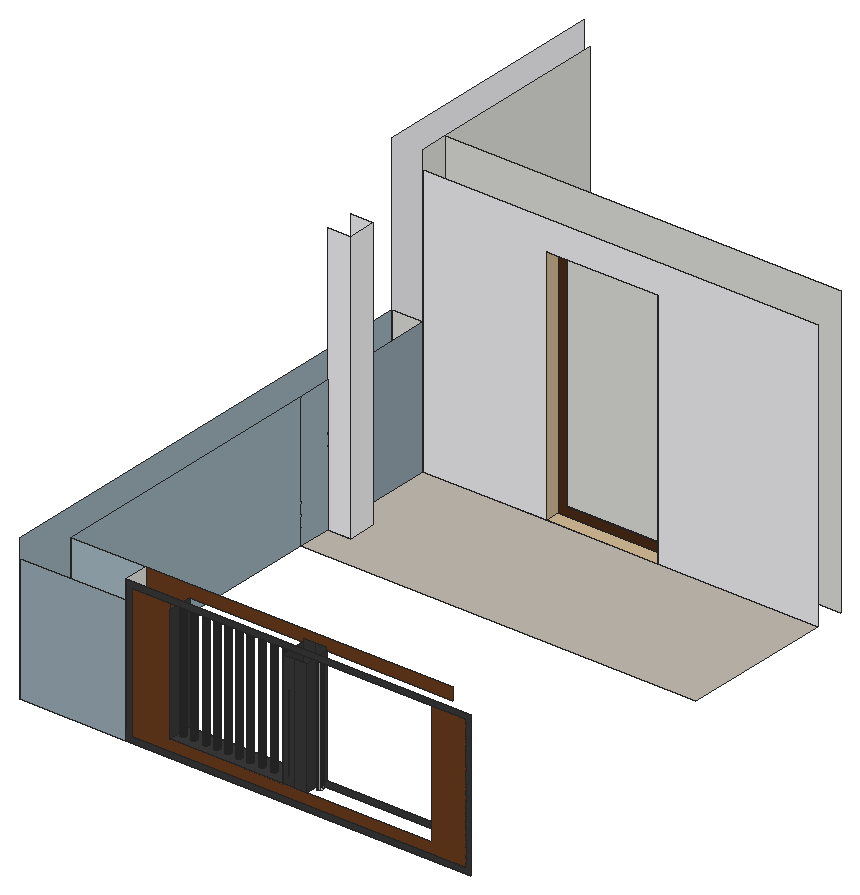
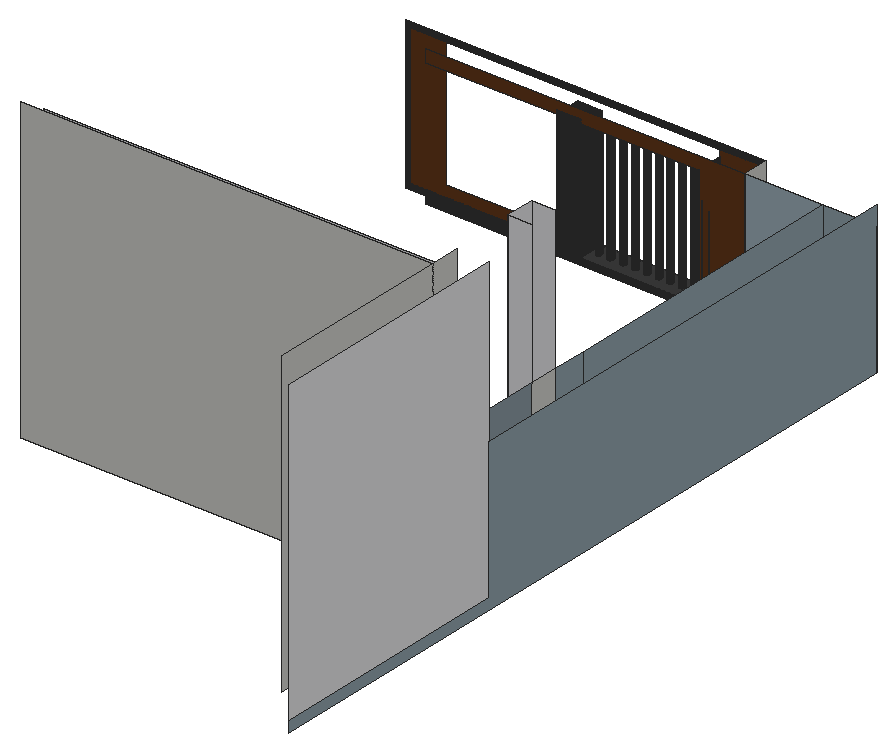
# SketchUp Ruby script. Lengths in inches.
U = 1.inch
M = Sketchup.active_model
def pt(a) = Geom::Point3d.new(a.map { |v| v * U })
def face(e, loops, mat)
  f = e.add_face(loops[0].map { |a| pt(a) })
  loops[1..].each { |l| e.add_face(l.map { |a| pt(a) }).erase! }
  f.material = f.back_material = mat if mat
  f
end
# faces: each face lists its corners as indices into pts; further lists are holes
def faces(e, pts, list, mat = nil) = list.each { |f| face(e, (f[0].is_a?(Array) ? f : [f]).map { |l| l.map { |i| pts[i] } }, mat) }
# xy, xz, yz: faces in a plane at the given z, y or x. An outline is a flat list of corners, or four numbers for a rectangle; further outlines are holes
def ring(l) = l.size == 4 ? [[l[0], l[1]], [l[2], l[1]], [l[2], l[3]], [l[0], l[3]]] : l.each_slice(2).to_a
def flat(e, list, mat, &to3) = list.each { |f| face(e, (f[0].is_a?(Array) ? f : [f]).map { |l| ring(l).map { |u, v| to3.(u, v) } }, mat) }
def xy(e, z, list, mat = nil) = flat(e, list, mat) { |x, y| [x, y, z] }
def xz(e, y, list, mat = nil) = flat(e, list, mat) { |x, z| [x, y, z] }
def yz(e, x, list, mat = nil) = flat(e, list, mat) { |y, z| [x, y, z] }
def lines(e, pts, list) = list.each { |a, b| e.add_line(pt(pts[a]), pt(pts[b])) }
# prism: a flat outline (further loops are holes) pulled along v
def prism(e, loops, v, mat = nil)
  f = face(e, loops, mat); d = Geom::Vector3d.new(v.map { |x| x * U })
  f.pushpull(f.normal.samedirection?(d) ? d.length : -d.length)
end
def box(e, o, s, mat = nil) = prism(e, [[o, [o[0] + s[0], o[1], o[2]], [o[0] + s[0], o[1] + s[1], o[2]], [o[0], o[1] + s[1], o[2]]]], [0, 0, s[2]], mat)
def at(x, y, z, deg = 0) = Geom::Transformation.translation(pt([x, y, z])) * Geom::Transformation.rotation(ORIGIN, Z_AXIS, deg.degrees)
def axes(o, x, y, z) = Geom::Transformation.new([*x, 0, *y, 0, *z, 0, *pt(o).to_a, 1])
def part(name) = M.definitions.add(name)
# library, detail: a bought-in or finely detailed component or shape, given as its bounding box
def library(name, o, s) = part(name).tap { |d| box(d.entities, o, s) }
def detail(e, o, s) = box(e.add_group.entities, o, s)
def put(e, d, t, mat = nil) = e.add_instance(d, t).tap { |i| i.material = mat if mat }
def group(e, t, mat = nil) = e.add_group.tap { |g| g.transformation = t; g.material = mat if mat }.entities
root = M.entities
M.materials.add("[Blinds Vertical Pattern]").color = [245, 245, 247]
M.materials.add("[Blinds Vertical Pattern]3").color = [247, 247, 249]
M.materials.add("[Color M03]").color = [170, 170, 170]
M.materials.add("[Color M07]").color = [58, 58, 58]
M.materials.add("[Field Rectangle Tile]").color = [196, 189, 179]
M.materials.add("[Formica Beige]").color = [211, 187, 149]
M.materials.add("[Formica Speckled Grey]").color = [157, 176, 186]
M.materials.add("[Formica Speckled Grey]1").color = [149, 166, 175]
M.materials.add("[Formica Speckled Grey]2").color = [170, 190, 201]
M.materials.add("[Wood Cherry Original]").color = [107, 60, 29]
M.materials.add("[Wood Veneer 01]").color = [76, 44, 23]
xy(root,9,[[62.71,489.78,81.96,513.87]])
xy(root,9,[[62.71,461.03,399.08,461.03,399.08,590.55,62.71,590.55,62.71,513.87,81.96,513.87,81.96,489.78,62.71,489.78]],"[Field Rectangle Tile]")
xy(root,9,[[168.16,590.55,262.6,602.92]],"[Formica Beige]")
xy(root,14.25,[[260.48,195.25,270.29,216.53],[270.29,195.25,280.09,216.53],[167.65,202.87,167.05,202.95,166.49,203.18,166.01,203.55,165.64,204.03,165.41,204.58,165.33,205.18,165.41,205.78,165.64,206.34,166.01,206.82,166.49,207.18,167.05,207.42,167.65,207.49,168.24,207.42,168.8,207.18,169.28,206.82,169.65,206.34,169.88,205.78,169.96,205.18,169.88,204.58,169.65,204.03,169.28,203.55,168.8,203.18,168.24,202.95],[176.58,202.87,175.98,202.95,175.43,203.18,174.95,203.55,174.58,204.03,174.35,204.58,174.27,205.18,174.35,205.78,174.58,206.34,174.95,206.82,175.43,207.18,175.98,207.42,176.58,207.49,177.18,207.42,177.74,207.18,178.22,206.82,178.59,206.34,178.82,205.78,178.9,205.18,178.82,204.58,178.59,204.03,178.22,203.55,177.74,203.18,177.18,202.95],[186.9,202.87,186.3,202.95,185.74,203.18,185.26,203.55,184.89,204.03,184.66,204.58,184.58,205.18,184.66,205.78,184.89,206.34,185.26,206.82,185.74,207.18,186.3,207.42,186.9,207.49,187.49,207.42,188.05,207.18,188.53,206.82,188.9,206.34,189.13,205.78,189.21,205.18,189.13,204.58,188.9,204.03,188.53,203.55,188.05,203.18,187.49,202.95],
  [196.21,202.87,195.61,202.95,195.05,203.18,194.57,203.55,194.21,204.03,193.97,204.58,193.9,205.18,193.97,205.78,194.21,206.34,194.57,206.82,195.05,207.18,195.61,207.42,196.21,207.49,196.81,207.42,197.36,207.18,197.84,206.82,198.21,206.34,198.44,205.78,198.52,205.18,198.44,204.58,198.21,204.03,197.84,203.55,197.36,203.18,196.81,202.95],[205.65,202.87,205.05,202.95,204.49,203.18,204.01,203.55,203.64,204.03,203.41,204.58,203.33,205.18,203.41,205.78,203.64,206.34,204.01,206.82,204.49,207.18,205.05,207.42,205.65,207.49,206.24,207.42,206.8,207.18,207.28,206.82,207.65,206.34,207.88,205.78,207.96,205.18,207.88,204.58,207.65,204.03,207.28,203.55,206.8,203.18,206.24,202.95],[215.27,202.87,214.67,202.95,214.11,203.18,213.64,203.55,213.27,204.03,213.04,204.58,212.96,205.18,213.04,205.78,213.27,206.34,213.64,206.82,214.11,207.18,214.67,207.42,215.27,207.49,215.87,207.42,216.43,207.18,216.91,206.82,217.27,206.34,217.5,205.78,217.58,205.18,217.5,204.58,217.27,204.03,216.91,203.55,216.43,203.18,215.87,202.95],[224.83,202.87,224.23,202.95,223.68,203.18,223.2,203.55,222.83,204.03,222.6,204.58,222.52,205.18,222.6,205.78,222.83,206.34,223.2,206.82,223.68,207.18,224.23,207.42,224.83,207.49,225.43,207.42,225.99,207.18,226.47,206.82,226.84,206.34,227.07,205.78,227.15,205.18,227.07,204.58,226.84,204.03,226.47,203.55,225.99,203.18,225.43,202.95],[234.71,202.87,234.11,202.95,233.55,203.18,233.07,203.55,232.71,204.03,232.47,204.58,232.4,205.18,232.47,205.78,232.71,206.34,233.07,206.82,233.55,207.18,234.11,207.42,234.71,207.49,235.31,207.42,235.86,207.18,236.34,206.82,236.71,206.34,236.94,205.78,237.02,205.18,236.94,204.58,236.71,204.03,236.34,203.55,235.86,203.18,235.31,202.95],
  [245.08,202.87,244.48,202.95,243.93,203.18,243.45,203.55,243.08,204.03,242.85,204.58,242.77,205.18,242.85,205.78,243.08,206.34,243.45,206.82,243.93,207.18,244.48,207.42,245.08,207.49,245.68,207.42,246.24,207.18,246.72,206.82,247.09,206.34,247.32,205.78,247.4,205.18,247.32,204.58,247.09,204.03,246.72,203.55,246.24,203.18,245.68,202.95],[254.71,202.87,254.11,202.95,253.55,203.18,253.07,203.55,252.71,204.03,252.47,204.58,252.4,205.18,252.47,205.78,252.71,206.34,253.07,206.82,253.55,207.18,254.11,207.42,254.71,207.49,255.31,207.42,255.86,207.18,256.34,206.82,256.71,206.34,256.94,205.78,257.02,205.18,256.94,204.58,256.71,204.03,256.34,203.55,255.86,203.18,255.31,202.95],[283.71,202.87,283.11,202.95,282.55,203.18,282.07,203.55,281.71,204.03,281.47,204.58,281.4,205.18,281.47,205.78,281.71,206.34,282.07,206.82,282.55,207.18,283.11,207.42,283.71,207.49,284.31,207.42,284.86,207.18,285.34,206.82,285.71,206.34,285.94,205.78,286.02,205.18,285.94,204.58,285.71,204.03,285.34,203.55,284.86,203.18,284.31,202.95]])
xy(root,14.25,[[[163.91,195.25,260.48,216.53],[167.65,202.87,167.05,202.95,166.49,203.18,166.01,203.55,165.64,204.03,165.41,204.58,165.33,205.18,165.41,205.78,165.64,206.34,166.01,206.82,166.49,207.18,167.05,207.42,167.65,207.49,168.24,207.42,168.8,207.18,169.28,206.82,169.65,206.34,169.88,205.78,169.96,205.18,169.88,204.58,169.65,204.03,169.28,203.55,168.8,203.18,168.24,202.95],[254.71,202.87,254.11,202.95,253.55,203.18,253.07,203.55,252.71,204.03,252.47,204.58,252.4,205.18,252.47,205.78,252.71,206.34,253.07,206.82,253.55,207.18,254.11,207.42,254.71,207.49,255.31,207.42,255.86,207.18,256.34,206.82,256.71,206.34,256.94,205.78,257.02,205.18,256.94,204.58,256.71,204.03,256.34,203.55,255.86,203.18,255.31,202.95],[176.58,202.87,175.98,202.95,175.43,203.18,174.95,203.55,174.58,204.03,174.35,204.58,174.27,205.18,174.35,205.78,174.58,206.34,174.95,206.82,175.43,207.18,175.98,207.42,176.58,207.49,177.18,207.42,177.74,207.18,178.22,206.82,178.59,206.34,178.82,205.78,178.9,205.18,178.82,204.58,178.59,204.03,178.22,203.55,177.74,203.18,177.18,202.95],[245.08,202.87,244.48,202.95,243.93,203.18,243.45,203.55,243.08,204.03,242.85,204.58,242.77,205.18,242.85,205.78,243.08,206.34,243.45,206.82,243.93,207.18,244.48,207.42,245.08,207.49,245.68,207.42,246.24,207.18,246.72,206.82,247.09,206.34,247.32,205.78,247.4,205.18,247.32,204.58,247.09,204.03,246.72,203.55,246.24,203.18,245.68,202.95],[186.9,202.87,186.3,202.95,185.74,203.18,185.26,203.55,184.89,204.03,184.66,204.58,184.58,205.18,184.66,205.78,184.89,206.34,185.26,206.82,185.74,207.18,186.3,207.42,186.9,207.49,187.49,207.42,188.05,207.18,188.53,206.82,188.9,206.34,189.13,205.78,189.21,205.18,189.13,204.58,188.9,204.03,188.53,203.55,188.05,203.18,187.49,202.95],[234.71,202.87,234.11,202.95,233.55,203.18,233.07,203.55,232.71,204.03,232.47,204.58,232.4,205.18,232.47,205.78,232.71,206.34,233.07,206.82,233.55,207.18,234.11,207.42,234.71,207.49,235.31,207.42,235.86,207.18,236.34,206.82,236.71,206.34,236.94,205.78,237.02,205.18,236.94,204.58,236.71,204.03,236.34,203.55,235.86,203.18,235.31,202.95],[196.21,202.87,195.61,202.95,195.05,203.18,194.57,203.55,194.21,204.03,193.97,204.58,193.9,205.18,193.97,205.78,194.21,206.34,194.57,206.82,195.05,207.18,195.61,207.42,196.21,207.49,196.81,207.42,197.36,207.18,197.84,206.82,198.21,206.34,198.44,205.78,198.52,205.18,198.44,204.58,198.21,204.03,197.84,203.55,197.36,203.18,196.81,202.95],[224.83,202.87,224.23,202.95,223.68,203.18,223.2,203.55,222.83,204.03,222.6,204.58,222.52,205.18,222.6,205.78,222.83,206.34,223.2,206.82,223.68,207.18,224.23,207.42,224.83,207.49,225.43,207.42,225.99,207.18,226.47,206.82,226.84,206.34,227.07,205.78,227.15,205.18,227.07,204.58,226.84,204.03,226.47,203.55,225.99,203.18,225.43,202.95],[205.65,202.87,205.05,202.95,204.49,203.18,204.01,203.55,203.64,204.03,203.41,204.58,203.33,205.18,203.41,205.78,203.64,206.34,204.01,206.82,204.49,207.18,205.05,207.42,205.65,207.49,206.24,207.42,206.8,207.18,207.28,206.82,207.65,206.34,207.88,205.78,207.96,205.18,207.88,204.58,207.65,204.03,207.28,203.55,206.8,203.18,206.24,202.95],[215.27,202.87,214.67,202.95,214.11,203.18,213.64,203.55,213.27,204.03,213.04,204.58,212.96,205.18,213.04,205.78,213.27,206.34,213.64,206.82,214.11,207.18,214.67,207.42,215.27,207.49,215.87,207.42,216.43,207.18,216.91,206.82,217.27,206.34,217.5,205.78,217.58,205.18,217.5,204.58,217.27,204.03,216.91,203.55,216.43,203.18,215.87,202.95]]],"[Color M07]")
xz(root,195.25,[[[126.39,0,420.08,122.8125],[131.23,4.5,416.17,118.1875]],[260.48,14.25,270.29,112.6],[270.29,14.25,280.09,112.6]],"[Color M07]")
xz(root,195.25,[[36.42,0,126.39,107.15]],"[Formica Speckled Grey]")
xz(root,195.25,[[131.23,4.5,416.17,4.5,416.17,118.1875,387.25,118.1875,387.25,14.25,163.91,14.25,163.91,118.1875,131.23,118.1875]],"[Wood Cherry Original]")
xz(root,216.53,[[163.91,9,387.25,14.25],[260.48,14.25,270.29,115.66],[270.29,14.25,280.09,115.66]],"[Color M07]")
xz(root,216.53,[[62.71,9,126.39,122.8125]],"[Formica Speckled Grey]2")
xz(root,216.53,[[126.39,9,126.39,122.8125,387.25,122.8125,387.25,112.6,280.09,112.6,280.09,115.66,260.48,115.66,260.48,112.6,163.91,112.6,163.91,9]],"[Wood Cherry Original]")
xz(root,489.78,[[62.71,9,81.96,238.875]],"[Blinds Vertical Pattern]")
xz(root,513.87,[[62.71,9,81.96,238.875]],"[Blinds Vertical Pattern]")
xz(root,590.55,[[36.42,9,62.71,122.8125]])
xz(root,590.55,[[62.71,9,168.16,9,168.16,213.75,262.6,213.75,262.6,9,399.08,9,399.08,238.875,62.71,238.875]],"[Blinds Vertical Pattern]")
xz(root,602.92,[[[168.16,9,262.6,213.75],[175.34,16.18,255.42,206.57]]],"[Wood Veneer 01]")
xz(root,614.75,[[62.71,9,399.08,254.375]])
yz(root,36.42,[[590.55,9,794.75,254.375]],"[Blinds Vertical Pattern]3")
yz(root,36.42,[[195.25,0,195.25,122.8125,590.55,122.8125,590.55,9,794.75,9,794.75,0]],"[Formica Speckled Grey]")
yz(root,62.71,[[489.78,9,513.87,122.8125],[590.55,9,614.75,254.375],[614.75,9,768.47,254.375]])
yz(root,62.71,[[216.53,9,461.03,122.8125],[461.03,9,489.78,122.8125]],"[Formica Speckled Grey]")
yz(root,62.71,[[513.87,9,590.55,122.8125]],"[Formica Speckled Grey]1")
yz(root,81.96,[[489.78,9,513.87,238.875]],"[Blinds Vertical Pattern]")
yz(root,126.39,[[195.25,9,216.53,122.8125]])
yz(root,163.91,[[195.25,14.25,216.53,112.6]],"[Color M07]")
yz(root,168.16,[[590.55,9,602.92,213.75]],"[Formica Beige]")
yz(root,260.48,[[195.25,14.25,216.53,112.6]],"[Color M07]")
yz(root,262.6,[[590.55,9,602.92,213.75]],"[Formica Beige]")
yz(root,280.09,[[195.25,14.25,216.53,112.6]],"[Color M07]")
p = [[166.49,203.18,14.25],[167.05,202.95,14.25],[167.05,202.95,112.6],[166.49,203.18,112.6],[167.65,202.87,14.25],[167.65,202.87,112.6],
  [168.24,202.95,14.25],[168.24,202.95,112.6],[168.8,203.18,14.25],[168.8,203.18,112.6],[175.43,203.18,14.25],[175.98,202.95,14.25],
  [175.98,202.95,112.6],[175.43,203.18,112.6],[176.58,202.87,14.25],[176.58,202.87,112.6],[177.18,202.95,14.25],[177.18,202.95,112.6],
  [177.74,203.18,14.25],[177.74,203.18,112.6],[185.74,203.18,14.25],[186.3,202.95,14.25],[186.3,202.95,112.6],[185.74,203.18,112.6],
  [186.9,202.87,14.25],[186.9,202.87,112.6],[187.49,202.95,14.25],[187.49,202.95,112.6],[188.05,203.18,14.25],[188.05,203.18,112.6],
  [195.05,203.18,14.25],[195.61,202.95,14.25],[195.61,202.95,112.6],[195.05,203.18,112.6],[196.21,202.87,14.25],[196.21,202.87,112.6],
  [196.81,202.95,14.25],[196.81,202.95,112.6],[197.36,203.18,14.25],[197.36,203.18,112.6],[204.49,203.18,14.25],[205.05,202.95,14.25],
  [205.05,202.95,112.6],[204.49,203.18,112.6],[205.65,202.87,14.25],[205.65,202.87,112.6],[206.24,202.95,14.25],[206.24,202.95,112.6],
  [206.8,203.18,14.25],[206.8,203.18,112.6],[214.11,203.18,14.25],[214.67,202.95,14.25],[214.67,202.95,112.6],[214.11,203.18,112.6],
  [215.27,202.87,14.25],[215.27,202.87,112.6],[215.87,202.95,14.25],[215.87,202.95,112.6],[216.43,203.18,14.25],[216.43,203.18,112.6],
  [223.68,203.18,14.25],[224.23,202.95,14.25],[224.23,202.95,112.6],[223.68,203.18,112.6],[224.83,202.87,14.25],[224.83,202.87,112.6],
  [225.43,202.95,14.25],[225.43,202.95,112.6],[225.99,203.18,14.25],[225.99,203.18,112.6],[233.55,203.18,14.25],[234.11,202.95,14.25],
  [234.11,202.95,112.6],[233.55,203.18,112.6],[234.71,202.87,14.25],[234.71,202.87,112.6],[235.31,202.95,14.25],[235.31,202.95,112.6],
  [235.86,203.18,14.25],[235.86,203.18,112.6],[243.93,203.18,14.25],[244.48,202.95,14.25],[244.48,202.95,112.6],[243.93,203.18,112.6],
  [245.08,202.87,14.25],[245.08,202.87,112.6],[245.68,202.95,14.25],[245.68,202.95,112.6],[246.24,203.18,14.25],[246.24,203.18,112.6],
  [253.55,203.18,14.25],[254.11,202.95,14.25],[254.11,202.95,112.6],[253.55,203.18,112.6],[254.71,202.87,14.25],[254.71,202.87,112.6],
  [255.31,202.95,14.25],[255.31,202.95,112.6],[255.86,203.18,14.25],[255.86,203.18,112.6],[282.55,203.18,14.25],[283.11,202.95,14.25],
  [283.11,202.95,112.6],[282.55,203.18,112.6],[283.71,202.87,14.25],[283.71,202.87,112.6],[284.31,202.95,14.25],[284.31,202.95,112.6],
  [284.86,203.18,14.25],[284.86,203.18,112.6],[166.01,203.55,14.25],[166.01,203.55,112.6],[169.28,203.55,14.25],[169.28,203.55,112.6],
  [174.95,203.55,14.25],[174.95,203.55,112.6],[178.22,203.55,14.25],[178.22,203.55,112.6],[185.26,203.55,14.25],[185.26,203.55,112.6],
  [188.53,203.55,14.25],[188.53,203.55,112.6],[194.57,203.55,14.25],[194.57,203.55,112.6],[197.84,203.55,14.25],[197.84,203.55,112.6],
  [204.01,203.55,14.25],[204.01,203.55,112.6],[207.28,203.55,14.25],[207.28,203.55,112.6],[213.64,203.55,14.25],[213.64,203.55,112.6],
  [216.91,203.55,14.25],[216.91,203.55,112.6],[223.2,203.55,14.25],[223.2,203.55,112.6],[226.47,203.55,14.25],[226.47,203.55,112.6],
  [233.07,203.55,14.25],[233.07,203.55,112.6],[236.34,203.55,14.25],[236.34,203.55,112.6],[243.45,203.55,14.25],[243.45,203.55,112.6],
  [246.72,203.55,14.25],[246.72,203.55,112.6],[253.07,203.55,14.25],[253.07,203.55,112.6],[256.34,203.55,14.25],[256.34,203.55,112.6],
  [282.07,203.55,14.25],[282.07,203.55,112.6],[165.64,204.03,14.25],[165.64,204.03,112.6],[169.65,204.03,14.25],[169.65,204.03,112.6],
  [174.58,204.03,14.25],[174.58,204.03,112.6],[178.59,204.03,14.25],[178.59,204.03,112.6],[184.89,204.03,14.25],[184.89,204.03,112.6],
  [188.9,204.03,14.25],[188.9,204.03,112.6],[194.21,204.03,14.25],[194.21,204.03,112.6],[198.21,204.03,14.25],[198.21,204.03,112.6],
  [203.64,204.03,14.25],[203.64,204.03,112.6],[207.65,204.03,14.25],[207.65,204.03,112.6],[213.27,204.03,14.25],[213.27,204.03,112.6],
  [217.27,204.03,14.25],[217.27,204.03,112.6],[222.83,204.03,14.25],[222.83,204.03,112.6],[226.84,204.03,14.25],[226.84,204.03,112.6],
  [232.71,204.03,14.25],[232.71,204.03,112.6],[236.71,204.03,14.25],[236.71,204.03,112.6],[243.08,204.03,14.25],[243.08,204.03,112.6],
  [247.09,204.03,14.25],[247.09,204.03,112.6],[252.71,204.03,14.25],[252.71,204.03,112.6],[256.71,204.03,14.25],[256.71,204.03,112.6],
  [281.71,204.03,14.25],[281.71,204.03,112.6],[165.41,204.58,14.25],[165.41,204.58,112.6],[169.88,204.58,14.25],[169.88,204.58,112.6],
  [174.35,204.58,14.25],[174.35,204.58,112.6],[178.82,204.58,14.25],[178.82,204.58,112.6],[184.66,204.58,14.25],[184.66,204.58,112.6],
  [189.13,204.58,14.25],[189.13,204.58,112.6],[193.97,204.58,14.25],[193.97,204.58,112.6],[198.44,204.58,14.25],[198.44,204.58,112.6],
  [203.41,204.58,14.25],[203.41,204.58,112.6],[207.88,204.58,14.25],[207.88,204.58,112.6],[213.04,204.58,14.25],[213.04,204.58,112.6],
  [217.5,204.58,14.25],[217.5,204.58,112.6],[222.6,204.58,14.25],[222.6,204.58,112.6],[227.07,204.58,14.25],[227.07,204.58,112.6],
  [232.47,204.58,14.25],[232.47,204.58,112.6],[236.94,204.58,14.25],[236.94,204.58,112.6],[242.85,204.58,14.25],[242.85,204.58,112.6],
  [247.32,204.58,14.25],[247.32,204.58,112.6],[252.47,204.58,14.25],[252.47,204.58,112.6],[256.94,204.58,14.25],[256.94,204.58,112.6],
  [281.47,204.58,14.25],[281.47,204.58,112.6],[165.33,205.18,14.25],[165.33,205.18,112.6],[169.96,205.18,14.25],[169.96,205.18,112.6],
  [174.27,205.18,14.25],[174.27,205.18,112.6],[178.9,205.18,14.25],[178.9,205.18,112.6],[184.58,205.18,14.25],[184.58,205.18,112.6],
  [189.21,205.18,14.25],[189.21,205.18,112.6],[193.9,205.18,14.25],[193.9,205.18,112.6],[198.52,205.18,14.25],[198.52,205.18,112.6],
  [203.33,205.18,14.25],[203.33,205.18,112.6],[207.96,205.18,14.25],[207.96,205.18,112.6],[212.96,205.18,14.25],[212.96,205.18,112.6],
  [217.58,205.18,14.25],[217.58,205.18,112.6],[222.52,205.18,14.25],[222.52,205.18,112.6],[227.15,205.18,14.25],[227.15,205.18,112.6],
  [232.4,205.18,14.25],[232.4,205.18,112.6],[237.02,205.18,14.25],[237.02,205.18,112.6],[242.77,205.18,14.25],[242.77,205.18,112.6],
  [247.4,205.18,14.25],[247.4,205.18,112.6],[252.4,205.18,14.25],[252.4,205.18,112.6],[257.02,205.18,14.25],[257.02,205.18,112.6],
  [281.4,205.18,14.25],[281.4,205.18,112.6],[165.41,205.78,14.25],[165.41,205.78,112.6],[169.88,205.78,14.25],[169.88,205.78,112.6],
  [174.35,205.78,14.25],[174.35,205.78,112.6],[178.82,205.78,14.25],[178.82,205.78,112.6],[184.66,205.78,14.25],[184.66,205.78,112.6],
  [189.13,205.78,14.25],[189.13,205.78,112.6],[193.97,205.78,14.25],[193.97,205.78,112.6],[198.44,205.78,14.25],[198.44,205.78,112.6],
  [203.41,205.78,14.25],[203.41,205.78,112.6],[207.88,205.78,14.25],[207.88,205.78,112.6],[213.04,205.78,14.25],[213.04,205.78,112.6],
  [217.5,205.78,14.25],[217.5,205.78,112.6],[222.6,205.78,14.25],[222.6,205.78,112.6],[227.07,205.78,14.25],[227.07,205.78,112.6],
  [232.47,205.78,14.25],[232.47,205.78,112.6],[236.94,205.78,14.25],[236.94,205.78,112.6],[242.85,205.78,14.25],[242.85,205.78,112.6],
  [247.32,205.78,14.25],[247.32,205.78,112.6],[252.47,205.78,14.25],[252.47,205.78,112.6],[256.94,205.78,14.25],[256.94,205.78,112.6],
  [281.47,205.78,14.25],[281.47,205.78,112.6],[165.64,206.34,14.25],[165.64,206.34,112.6],[169.65,206.34,14.25],[169.65,206.34,112.6],
  [174.58,206.34,14.25],[174.58,206.34,112.6],[178.59,206.34,14.25],[178.59,206.34,112.6],[184.89,206.34,14.25],[184.89,206.34,112.6],
  [188.9,206.34,14.25],[188.9,206.34,112.6],[194.21,206.34,14.25],[194.21,206.34,112.6],[198.21,206.34,14.25],[198.21,206.34,112.6],
  [203.64,206.34,14.25],[203.64,206.34,112.6],[207.65,206.34,14.25],[207.65,206.34,112.6],[213.27,206.34,14.25],[213.27,206.34,112.6],
  [217.27,206.34,14.25],[217.27,206.34,112.6],[222.83,206.34,14.25],[222.83,206.34,112.6],[226.84,206.34,14.25],[226.84,206.34,112.6],
  [232.71,206.34,14.25],[232.71,206.34,112.6],[236.71,206.34,14.25],[236.71,206.34,112.6],[243.08,206.34,14.25],[243.08,206.34,112.6],
  [247.09,206.34,14.25],[247.09,206.34,112.6],[252.71,206.34,14.25],[252.71,206.34,112.6],[256.71,206.34,14.25],[256.71,206.34,112.6],
  [281.71,206.34,14.25],[281.71,206.34,112.6],[166.01,206.82,14.25],[166.01,206.82,112.6],[169.28,206.82,14.25],[169.28,206.82,112.6],
  [174.95,206.82,14.25],[174.95,206.82,112.6],[178.22,206.82,14.25],[178.22,206.82,112.6],[185.26,206.82,14.25],[185.26,206.82,112.6],
  [188.53,206.82,14.25],[188.53,206.82,112.6],[194.57,206.82,14.25],[194.57,206.82,112.6],[197.84,206.82,14.25],[197.84,206.82,112.6],
  [204.01,206.82,14.25],[204.01,206.82,112.6],[207.28,206.82,14.25],[207.28,206.82,112.6],[213.64,206.82,14.25],[213.64,206.82,112.6],
  [216.91,206.82,14.25],[216.91,206.82,112.6],[223.2,206.82,14.25],[223.2,206.82,112.6],[226.47,206.82,14.25],[226.47,206.82,112.6],
  [233.07,206.82,14.25],[233.07,206.82,112.6],[236.34,206.82,14.25],[236.34,206.82,112.6],[243.45,206.82,14.25],[243.45,206.82,112.6],
  [246.72,206.82,14.25],[246.72,206.82,112.6],[253.07,206.82,14.25],[253.07,206.82,112.6],[256.34,206.82,14.25],[256.34,206.82,112.6],
  [282.07,206.82,14.25],[282.07,206.82,112.6],[166.49,207.18,14.25],[166.49,207.18,112.6],[168.8,207.18,14.25],[168.8,207.18,112.6],
  [175.43,207.18,14.25],[175.43,207.18,112.6],[177.74,207.18,14.25],[177.74,207.18,112.6],[185.74,207.18,14.25],[185.74,207.18,112.6],
  [188.05,207.18,14.25],[188.05,207.18,112.6],[195.05,207.18,14.25],[195.05,207.18,112.6],[197.36,207.18,14.25],[197.36,207.18,112.6],
  [204.49,207.18,14.25],[204.49,207.18,112.6],[206.8,207.18,14.25],[206.8,207.18,112.6],[214.11,207.18,14.25],[214.11,207.18,112.6],
  [216.43,207.18,14.25],[216.43,207.18,112.6],[223.68,207.18,14.25],[223.68,207.18,112.6],[225.99,207.18,14.25],[225.99,207.18,112.6],
  [233.55,207.18,14.25],[233.55,207.18,112.6],[235.86,207.18,14.25],[235.86,207.18,112.6],[243.93,207.18,14.25],[243.93,207.18,112.6],
  [246.24,207.18,14.25],[246.24,207.18,112.6],[253.55,207.18,14.25],[253.55,207.18,112.6],[255.86,207.18,14.25],[255.86,207.18,112.6],
  [282.55,207.18,14.25],[282.55,207.18,112.6],[285.34,206.82,14.25],[284.86,207.18,14.25],[284.86,207.18,112.6],[285.34,206.82,112.6],
  [167.05,207.42,14.25],[167.05,207.42,112.6],[168.24,207.42,14.25],[168.24,207.42,112.6],[175.98,207.42,14.25],[175.98,207.42,112.6],
  [177.18,207.42,14.25],[177.18,207.42,112.6],[186.3,207.42,14.25],[186.3,207.42,112.6],[187.49,207.42,14.25],[187.49,207.42,112.6],
  [195.61,207.42,14.25],[195.61,207.42,112.6],[196.81,207.42,14.25],[196.81,207.42,112.6],[205.05,207.42,14.25],[205.05,207.42,112.6],
  [206.24,207.42,14.25],[206.24,207.42,112.6],[214.67,207.42,14.25],[214.67,207.42,112.6],[215.87,207.42,14.25],[215.87,207.42,112.6],
  [224.23,207.42,14.25],[224.23,207.42,112.6],[225.43,207.42,14.25],[225.43,207.42,112.6],[234.11,207.42,14.25],[234.11,207.42,112.6],
  [235.31,207.42,14.25],[235.31,207.42,112.6],[244.48,207.42,14.25],[244.48,207.42,112.6],[245.68,207.42,14.25],[245.68,207.42,112.6],
  [254.11,207.42,14.25],[254.11,207.42,112.6],[255.31,207.42,14.25],[255.31,207.42,112.6],[283.11,207.42,14.25],[283.11,207.42,112.6],
  [284.31,207.42,14.25],[284.31,207.42,112.6],[167.65,207.49,14.25],[167.65,207.49,112.6],[176.58,207.49,14.25],[176.58,207.49,112.6],
  [186.9,207.49,14.25],[186.9,207.49,112.6],[196.21,207.49,14.25],[196.21,207.49,112.6],[205.65,207.49,14.25],[205.65,207.49,112.6],
  [215.27,207.49,14.25],[215.27,207.49,112.6],[224.83,207.49,14.25],[224.83,207.49,112.6],[234.71,207.49,14.25],[234.71,207.49,112.6],
  [245.08,207.49,14.25],[245.08,207.49,112.6],[254.71,207.49,14.25],[254.71,207.49,112.6],[283.71,207.49,14.25],[283.71,207.49,112.6]]
faces(root,p,[[0,1,2,3],[1,4,5,2],[4,6,7,5],[6,8,9,7],[10,11,12,13],[11,14,15,12],[14,16,17,15],[16,18,19,17],
  [20,21,22,23],[21,24,25,22],[24,26,27,25],[26,28,29,27],[30,31,32,33],[31,34,35,32],[34,36,37,35],[36,38,39,37],
  [40,41,42,43],[41,44,45,42],[44,46,47,45],[46,48,49,47],[50,51,52,53],[51,54,55,52],[54,56,57,55],[56,58,59,57],
  [60,61,62,63],[61,64,65,62],[64,66,67,65],[66,68,69,67],[70,71,72,73],[71,74,75,72],[74,76,77,75],[76,78,79,77],
  [80,81,82,83],[81,84,85,82],[84,86,87,85],[86,88,89,87],[90,91,92,93],[91,94,95,92],[94,96,97,95],[96,98,99,97],
  [100,101,102,103],[101,104,105,102],[104,106,107,105],[106,108,109,107],[110,0,3,111],[8,112,113,9],[114,10,13,115],[18,116,117,19],
  [118,20,23,119],[28,120,121,29],[122,30,33,123],[38,124,125,39],[126,40,43,127],[48,128,129,49],[130,50,53,131],[58,132,133,59],
  [134,60,63,135],[68,136,137,69],[138,70,73,139],[78,140,141,79],[142,80,83,143],[88,144,145,89],[146,90,93,147],[98,148,149,99],
  [150,100,103,151],[152,110,111,153],[112,154,155,113],[156,114,115,157],[116,158,159,117],[160,118,119,161],[120,162,163,121],[164,122,123,165],
  [124,166,167,125],[168,126,127,169],[128,170,171,129],[172,130,131,173],[132,174,175,133],[176,134,135,177],[136,178,179,137],[180,138,139,181],
  [140,182,183,141],[184,142,143,185],[144,186,187,145],[188,146,147,189],[148,190,191,149],[192,150,151,193],[194,152,153,195],[154,196,197,155],
  [198,156,157,199],[158,200,201,159],[202,160,161,203],[162,204,205,163],[206,164,165,207],[166,208,209,167],[210,168,169,211],[170,212,213,171],
  [214,172,173,215],[174,216,217,175],[218,176,177,219],[178,220,221,179],[222,180,181,223],[182,224,225,183],[226,184,185,227],[186,228,229,187],
  [230,188,189,231],[190,232,233,191],[234,192,193,235],[236,194,195,237],[196,238,239,197],[240,198,199,241],[200,242,243,201],[244,202,203,245],
  [204,246,247,205],[248,206,207,249],[208,250,251,209],[252,210,211,253],[212,254,255,213],[256,214,215,257],[216,258,259,217],[260,218,219,261],
  [220,262,263,221],[264,222,223,265],[224,266,267,225],[268,226,227,269],[228,270,271,229],[272,230,231,273],[232,274,275,233],[276,234,235,277],
  [278,236,237,279],[238,280,281,239],[282,240,241,283],[242,284,285,243],[286,244,245,287],[246,288,289,247],[290,248,249,291],[250,292,293,251],
  [294,252,253,295],[254,296,297,255],[298,256,257,299],[258,300,301,259],[302,260,261,303],[262,304,305,263],[306,264,265,307],[266,308,309,267],
  [310,268,269,311],[270,312,313,271],[314,272,273,315],[274,316,317,275],[318,276,277,319],[320,278,279,321],[280,322,323,281],[324,282,283,325],
  [284,326,327,285],[328,286,287,329],[288,330,331,289],[332,290,291,333],[292,334,335,293],[336,294,295,337],[296,338,339,297],[340,298,299,341],
  [300,342,343,301],[344,302,303,345],[304,346,347,305],[348,306,307,349],[308,350,351,309],[352,310,311,353],[312,354,355,313],[356,314,315,357],
  [316,358,359,317],[360,318,319,361],[362,320,321,363],[322,364,365,323],[366,324,325,367],[326,368,369,327],[370,328,329,371],[330,372,373,331],
  [374,332,333,375],[334,376,377,335],[378,336,337,379],[338,380,381,339],[382,340,341,383],[342,384,385,343],[386,344,345,387],[346,388,389,347],
  [390,348,349,391],[350,392,393,351],[394,352,353,395],[354,396,397,355],[398,356,357,399],[358,400,401,359],[402,360,361,403],[404,362,363,405],
  [364,406,407,365],[408,366,367,409],[368,410,411,369],[412,370,371,413],[372,414,415,373],[416,374,375,417],[376,418,419,377],[420,378,379,421],
  [380,422,423,381],[424,382,383,425],[384,426,427,385],[428,386,387,429],[388,430,431,389],[432,390,391,433],[392,434,435,393],[436,394,395,437],
  [396,438,439,397],[440,398,399,441],[400,442,443,401],[444,402,403,445],[446,447,448,449],[450,404,405,451],[406,452,453,407],[454,408,409,455],
  [410,456,457,411],[458,412,413,459],[414,460,461,415],[462,416,417,463],[418,464,465,419],[466,420,421,467],[422,468,469,423],[470,424,425,471],
  [426,472,473,427],[474,428,429,475],[430,476,477,431],[478,432,433,479],[434,480,481,435],[482,436,437,483],[438,484,485,439],[486,440,441,487],
  [442,488,489,443],[490,444,445,491],[447,492,493,448],[494,450,451,495],[452,494,495,453],[496,454,455,497],[456,496,497,457],[498,458,459,499],
  [460,498,499,461],[500,462,463,501],[464,500,501,465],[502,466,467,503],[468,502,503,469],[504,470,471,505],[472,504,505,473],[506,474,475,507],
  [476,506,507,477],[508,478,479,509],[480,508,509,481],[510,482,483,511],[484,510,511,485],[512,486,487,513],[488,512,513,489],[514,490,491,515],
  [492,514,515,493]],"[Color M03]")
